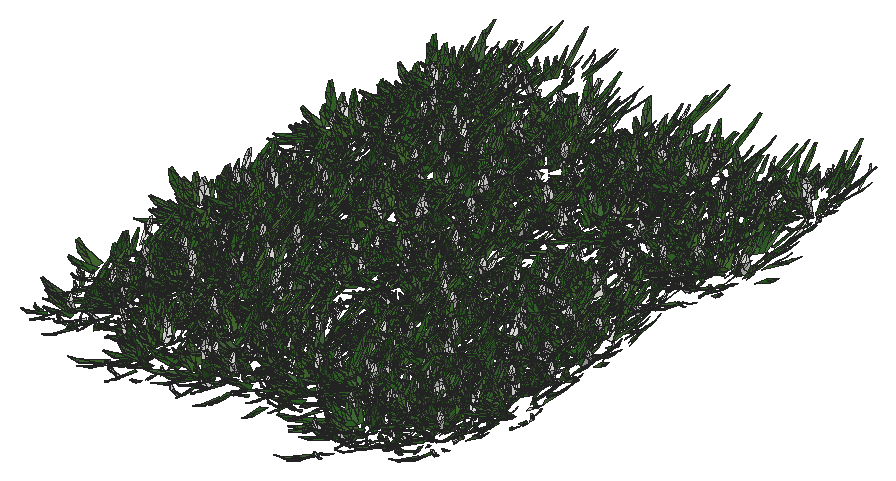
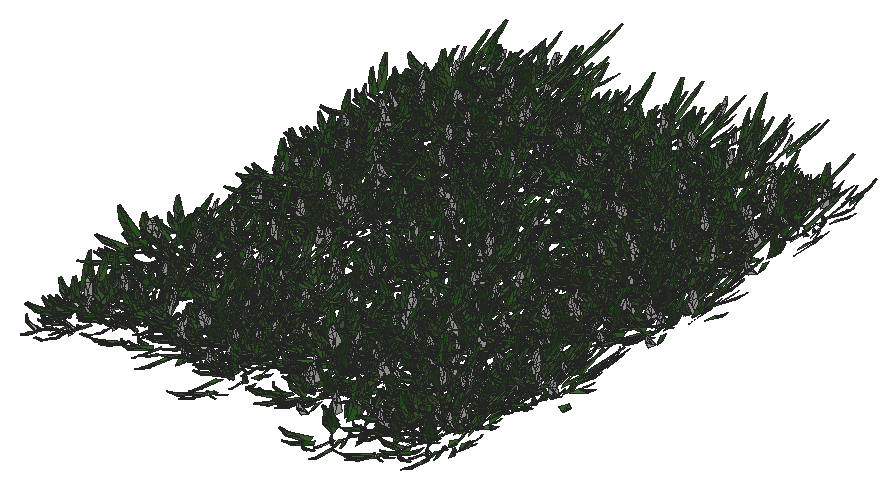
# SketchUp Ruby script. Lengths in inches.
U = 1.inch
M = Sketchup.active_model
def pt(a) = Geom::Point3d.new(a.map { |v| v * U })
def face(e, loops, mat)
  f = e.add_face(loops[0].map { |a| pt(a) })
  loops[1..].each { |l| e.add_face(l.map { |a| pt(a) }).erase! }
  f.material = f.back_material = mat if mat
  f
end
# faces: each face lists its corners as indices into pts; further lists are holes
def faces(e, pts, list, mat = nil) = list.each { |f| face(e, (f[0].is_a?(Array) ? f : [f]).map { |l| l.map { |i| pts[i] } }, mat) }
# xy, xz, yz: faces in a plane at the given z, y or x. An outline is a flat list of corners, or four numbers for a rectangle; further outlines are holes
def ring(l) = l.size == 4 ? [[l[0], l[1]], [l[2], l[1]], [l[2], l[3]], [l[0], l[3]]] : l.each_slice(2).to_a
def flat(e, list, mat, &to3) = list.each { |f| face(e, (f[0].is_a?(Array) ? f : [f]).map { |l| ring(l).map { |u, v| to3.(u, v) } }, mat) }
def xy(e, z, list, mat = nil) = flat(e, list, mat) { |x, y| [x, y, z] }
def xz(e, y, list, mat = nil) = flat(e, list, mat) { |x, z| [x, y, z] }
def yz(e, x, list, mat = nil) = flat(e, list, mat) { |y, z| [x, y, z] }
def lines(e, pts, list) = list.each { |a, b| e.add_line(pt(pts[a]), pt(pts[b])) }
# prism: a flat outline (further loops are holes) pulled along v
def prism(e, loops, v, mat = nil)
  f = face(e, loops, mat); d = Geom::Vector3d.new(v.map { |x| x * U })
  f.pushpull(f.normal.samedirection?(d) ? d.length : -d.length)
end
def box(e, o, s, mat = nil) = prism(e, [[o, [o[0] + s[0], o[1], o[2]], [o[0] + s[0], o[1] + s[1], o[2]], [o[0], o[1] + s[1], o[2]]]], [0, 0, s[2]], mat)
def at(x, y, z, deg = 0) = Geom::Transformation.translation(pt([x, y, z])) * Geom::Transformation.rotation(ORIGIN, Z_AXIS, deg.degrees)
def axes(o, x, y, z) = Geom::Transformation.new([*x, 0, *y, 0, *z, 0, *pt(o).to_a, 1])
def part(name) = M.definitions.add(name)
# library, detail: a bought-in or finely detailed component or shape, given as its bounding box
def library(name, o, s) = part(name).tap { |d| box(d.entities, o, s) }
def detail(e, o, s) = box(e.add_group.entities, o, s)
def put(e, d, t, mat = nil) = e.add_instance(d, t).tap { |i| i.material = mat if mat }
def group(e, t, mat = nil) = e.add_group.tap { |g| g.transformation = t; g.material = mat if mat }.entities
root = M.entities
M.materials.add("Material10").color = [48, 90, 38]
M.materials.add("Material11").color = [68, 110, 48]
M.materials.add("Material12").color = [48, 90, 48]
M.materials.add("Material13").color = [58, 110, 58]
M.materials.add("Material14").color = [58, 90, 38]
M.materials.add("Material15").color = [68, 100, 58]
M.materials.add("Material16").color = [48, 100, 38]
M.materials.add("Material9").color = [68, 110, 58]
c1 = part("grass00")
p = [[-0.6875,0.15,0],[-0.56,0.08,5.52],[-0.04,0.03,2.76],[0.48,-0.02,0],[0.35,-0.02,5.52],[-0.1,-0.14,5.52],
  [-0.12,0.65,8.37],[-0.42,0.65,8.37]]
faces(c1.entities,p,[[0,1,2,3],[3,2,4],[1,5,2],[5,4,2],[1,6,5],[4,5,6],[7,6,1]])
c2 = part("Group16\#1")
put(c2.entities,c1,axes([1.44,-0.61,-0.01],[0.05352,0.12609,0],[-0.10704,0.04543,0.07239],[0.06664,-0.02828,0.11628]),"Material12")
put(c2.entities,c1,axes([0.76,-0.15,-0.01],[0.04676,0.24062,0],[-0.23162,0.04501,0.06642],[0.0652,-0.01267,0.23595]),"Material9")
put(c2.entities,c1,axes([0.79,0.01,-0.01],[-0.00606,0.34651,0],[-0.34381,-0.00602,0.0432],[0.04319,0.00076,0.34386]))
put(c2.entities,c1,axes([1,0.23,-0.01],[-0.07192,0.31144,0],[-0.28722,-0.06632,0.1236],[0.12043,0.02781,0.29478]),"Material11")
put(c2.entities,c1,axes([1.66,0.77,-0.01],[-0.13828,0.29651,0],[-0.21551,-0.1005,0.22471],[0.20365,0.09498,0.23779]),"Material16")
put(c2.entities,c1,axes([0.6875,0.52,-0.01],[-0.18126,0.24051,0],[-0.22746,-0.17142,0.09788],[0.07817,0.05891,0.28481]),"Material11")
put(c2.entities,c1,axes([0.68,0.78,-0.01],[-0.215,0.18688,0],[-0.12385,-0.14248,0.21334],[0.13995,0.16101,0.18878]),"Material9")
put(c2.entities,c1,axes([0.56,1,-0.01],[-0.13756,0.07624,0],[-0.06159,-0.11112,0.0927],[0.04494,0.08108,0.12705]),"Material11")
put(c2.entities,c1,axes([0.2,0.64,-0.01],[-0.23729,0.07254,0],[-0.05711,-0.18681,0.153],[0.04473,0.14632,0.19535]),"Material16")
put(c2.entities,c1,axes([0.0625,0.72,-0.01],[-0.28874,0.02525,0],[-0.02179,-0.24916,0.14647],[0.01276,0.14591,0.25012]),"Material9")
put(c2.entities,c1,axes([-0.08,0.62,-0.01],[-0.34089,-0.04187,0],[0.03255,-0.26504,0.216],[-0.02633,0.21439,0.26703]),"Material16")
put(c2.entities,c1,axes([-0.34,0.98,-0.01],[-0.14314,-0.0493,0],[0.04397,-0.12769,0.06843],[-0.02228,0.0647,0.13505]),"Material16")
put(c2.entities,c1,axes([-0.87,1.45,-0.01],[-0.23488,-0.14114,0],[0.13761,-0.22901,0.06087],[-0.03135,0.05217,0.26717]))
put(c2.entities,c1,axes([-0.72,0.77,-0.01],[-0.14208,-0.13251,0],[0.07209,-0.0773,0.16301],[-0.11118,0.11922,0.1057]),"Material16")
put(c2.entities,c1,axes([-0.62,0.43,-0.01],[-0.14845,-0.21203,0],[0.18654,-0.13061,0.12304],[-0.10079,0.07057,0.22772]),"Material9")
put(c2.entities,c1,axes([-0.68,0.29,-0.01],[-0.13639,-0.32136,0],[0.31723,-0.13464,0.05579],[-0.05136,0.0218,0.34462]),"Material10")
put(c2.entities,c1,axes([-0.64,0.125,-0.01],[-0.0458,-0.23569,0],[0.22124,-0.043,0.08276],[-0.08124,0.01579,0.22538]),"Material13")
put(c2.entities,c1,axes([-1.6,-0.03,-0.01],[0.00576,-0.32897,0],[0.27526,0.00482,0.18018],[-0.18015,-0.00315,0.2753]),"Material11")
put(c2.entities,c1,axes([-1.36,-0.31,-0.01],[0.05718,-0.24765,0],[0.18172,0.04196,0.17267],[-0.16825,-0.03885,0.1865]),"Material16")
put(c2.entities,c1,axes([-1.54,-0.72,-0.01],[0.06537,-0.14017,0],[0.13555,0.06321,0.03939],[-0.0357,-0.01665,0.14956]))
put(c2.entities,c1,axes([-1.19,-0.9,-0.01],[0.09597,-0.12735,0],[0.11214,0.08451,0.07557],[-0.06035,-0.04548,0.14042]),"Material15")
put(c2.entities,c1,axes([-0.47,-0.54,-0.01],[0.11588,-0.10072,0],[0.0618,0.0711,0.12124],[-0.07953,-0.0915,0.0942]))
put(c2.entities,c1,axes([-0.47,-0.84,-0.01],[0.11927,-0.0661,0],[0.06603,0.11913,0.00646],[-0.00313,-0.00565,0.13621]),"Material11")
put(c2.entities,c1,axes([-0.38,-1.24,-0.01],[0.28037,-0.08571,0],[0.0618,0.20215,0.20315],[-0.05939,-0.19428,0.21139]),"Material15")
put(c2.entities,c1,axes([-0.06,-0.66,-0.01],[0.22719,-0.01987,0],[0.01247,0.14255,0.17758],[-0.01547,-0.17691,0.1431]),"Material14")
put(c2.entities,c1,axes([0.11,-0.89,-0.01],[0.14882,0.01828,0],[-0.01058,0.08611,0.12229],[0.01491,-0.12138,0.08676]),"Material12")
put(c2.entities,c1,axes([0.25,-0.72,-0.01],[0.20481,0.07053,0],[-0.06206,0.18022,0.10291],[0.03351,-0.0973,0.1906]),"Material12")
put(c2.entities,c1,axes([0.85,-1.42,-0.01],[0.16481,0.09904,0],[-0.09472,0.15762,0.05616],[0.02893,-0.04814,0.18389]),"Material11")
put(c2.entities,c1,axes([1.01,-1.09,-0.01],[0.21858,0.20385,0],[-0.17495,0.1876,0.15339],[0.10462,-0.11218,0.25652]),"Material16")
put(c2.entities,c1,axes([1.01,-0.71,-0.01],[0.08733,0.12473,0],[-0.06445,0.04512,0.13037],[0.1068,-0.07477,0.07867]),"Material12")
c3 = part("Group15\#1")
put(c3.entities,c2,at(0,0,0))
c4 = part("3darcstudiotree_grass00\#1")
put(c4.entities,c3,at(0,0,0))
put(root,c4,axes([827.38,626.97,12.99],[-2.37423,5.49168,0],[-1.9202,-4.33781,-0.03007],[-0.11385,-0.2572,1.97134]))
put(root,c4,axes([873.03,627.38,12.99],[0.43076,7.5469,0],[-2.49885,0.74527,-0.03746],[-0.18093,0.05396,1.68385]))
put(root,c4,axes([877.48,630.32,12.99],[2.41678,2.99983,0],[-1.2331,5.19091,-0.03457],[-0.08948,0.37667,1.92264]))
put(root,c4,axes([838.15,629.06,12.99],[-2.83663,1.42991,0],[-0.68383,-7.08843,-0.02531],[-0.02216,-0.2297,1.77094]))
put(root,c4,axes([824.06,630.47,12.99],[1.45141,7.05761,0],[-2.63622,2.83281,-0.03464],[-0.13976,0.15018,1.78143]))
put(root,c4,axes([851.625,633.5,12.99],[-0.02714,-5.82312,0],[3.4571,-0.0842,-0.05216],[0.14988,-0.00365,1.36288]))
put(root,c4,axes([803.71,634.1,12.99],[0.90647,-5.26217,0],[2.79568,2.51641,-0.0431],[0.13449,0.12105,1.38217]))
put(root,c4,axes([808.97,633.48,12.99],[2.65153,2.38197,0],[-1.03238,6.00489,-0.02634],[-0.03943,0.22937,1.58474]))
put(root,c4,axes([842.07,635.41,12.99],[0.95151,-7.55802,0],[3.30412,2.17354,-0.04991],[0.1976,0.12999,1.94306]))
put(root,c4,axes([870.84,632.96,12.99],[-3.13855,-0.88162,0],[0.39114,-7.27583,-0.04768],[0.0198,-0.36827,1.49744]))
put(root,c4,axes([843.74,633.08,12.99],[-1.41677,7.11189,0],[-2.22403,-2.31505,-0.04508],[-0.16224,-0.16888,1.32557]))
put(root,c4,axes([824.7,635.18,12.99],[-0.89079,-5.45923,0],[2.93999,-2.50666,-0.0406],[0.16325,-0.13919,1.84742]))
put(root,c4,axes([882.71,635.9,12.99],[2.96033,-0.5202,0],[0.24057,7.15334,-0.03486],[0.01046,0.311,1.68524]))
put(root,c4,axes([836.04,637.33,12.99],[0.52554,-6.14252,0],[3.42043,1.52912,-0.06032],[0.17465,0.07808,1.41053]))
put(root,c4,axes([820.39,637.29,12.99],[0.17649,-6.6496,0],[3.22338,0.44704,-0.04584],[0.13578,0.01883,1.3146]))
put(root,c4,axes([861.75,637.18,12.99],[2.53106,4.3429,0],[-1.85243,5.64117,-0.02233],[-0.06236,0.18989,1.9689]))
put(root,c4,axes([856.68,636.47,12.99],[-2.58773,4.03605,0],[-1.59912,-5.35732,-0.04776],[-0.11569,-0.38757,1.6727]))
put(root,c4,axes([874.8125,638.46,12.99],[1.38554,6.71769,0],[-2.60751,2.81016,-0.03917],[-0.16088,0.17338,1.79585]))
put(root,c4,axes([866.72,638.83,12.99],[0.12549,7.79346,0],[-3.40251,0.28627,-0.03073],[-0.09784,0.00823,1.48809]))
put(root,c4,axes([886.75,638.65,12.99],[-0.79908,7.12585,0],[-3.17807,-1.86218,-0.05431],[-0.19695,-0.1154,1.6847]))
put(root,c4,axes([836.7,642.28,12.99],[2.73963,-0.34023,0],[0.14501,6.10118,-0.02262],[0.0054,0.22718,1.6131]))
put(root,c4,axes([811.9,639.8,12.99],[-1.74597,5.76407,0],[-2.15705,-3.41407,-0.03104],[-0.12661,-0.20039,1.78553]))
put(root,c4,axes([851.64,642.82,12.99],[-0.39937,-7.02713,0],[2.45826,-0.73001,-0.04034],[0.17351,-0.05153,1.47504]))
put(root,c4,axes([832.96,643.67,12.99],[-1.43376,-4.96537,0],[2.07832,-3.13575,-0.03406],[0.14408,-0.21739,1.73123]))
put(root,c4,axes([862.18,644.98,12.99],[2.57457,-3.51757,0],[1.66433,6.36512,-0.05659],[0.10752,0.4112,1.64805]))
put(root,c4,axes([810.82,642.92,12.99],[-2.82662,-1.37215,0],[0.64948,-6.99095,-0.02543],[0.0198,-0.2131,1.60712]))
put(root,c4,axes([847.42,645.02,12.99],[-0.04441,-5.91504,0],[3.02597,-0.11872,-0.0405],[0.18434,-0.00723,1.89003]))
put(root,c4,axes([881.23,642.45,12.99],[-3.19545,2.75579,0],[-1.21799,-7.37964,-0.03096],[-0.04152,-0.25159,1.79846]))
put(root,c4,axes([846.15,643.85,12.99],[-0.34531,6.17385,0],[-3.32473,-0.97165,-0.0277],[-0.11233,-0.03283,1.87956]))
put(root,c4,axes([878.14,645.06,12.99],[1.84367,4.1672,0],[-1.70839,3.94941,-0.02576],[-0.1024,0.23673,1.88472]))
put(root,c4,axes([825.89,648.15,12.99],[1.25304,-5.40337,0],[2.85201,3.45587,-0.01977],[0.07044,0.08535,1.78562]))
put(root,c4,axes([886.66,647,12.99],[1.945,3.95778,0],[-2.10927,5.41631,-0.03405],[-0.08629,0.22159,1.65877]))
put(root,c4,axes([802.61,648.01,12.99],[3.06395,1.36265,0],[-0.61914,7.27433,-0.03864],[-0.03074,0.36119,1.85268]))
put(root,c4,axes([809.37,648.66,12.99],[2.23298,-4.95504,0],[1.79016,4.21537,-0.02978],[0.08432,0.19856,1.43312]))
put(root,c4,axes([857.9375,647.72,12.99],[-1.4711,-5.8297,0],[2.67186,-3.52304,-0.05686],[0.15267,-0.2013,1.31145]))
put(root,c4,axes([815.91,646.11,12.99],[-0.90996,6.13703,0],[-2.95759,-2.29145,-0.05878],[-0.18054,-0.13988,1.38915]))
put(root,c4,axes([868.14,647.99,12.99],[-2.61801,-2.5298,0],[1.19759,-6.4759,-0.0473],[0.06262,-0.3386,1.43445]))
put(root,c4,axes([865.81,649.17,12.99],[2.88934,4.27674,0],[-1.72566,6.09181,-0.02279],[-0.05355,0.18905,1.88252]))
put(root,c4,axes([845.39,653.56,12.99],[-0.34485,-6.99494,0],[2.81083,-0.72408,-0.02839],[0.09584,-0.02469,1.31807]))
put(root,c4,axes([876.6,652.99,12.99],[-1.44959,-4.55091,0],[2.53951,-4.22671,-0.06067],[0.206,-0.34286,1.80988]))
put(root,c4,axes([890.19,652.17,12.99],[-2.81566,3.68421,0],[-1.29367,-5.16611,-0.03218],[-0.07418,-0.29624,1.65786]))
put(root,c4,axes([856.61,653.59,12.99],[1.64625,5.68783,0],[-2.83649,4.28977,-0.02773],[-0.07489,0.11325,1.51065]))
put(root,c4,axes([864.83,652.91,12.99],[1.37491,7.18474,0],[-2.38597,2.3858,-0.02724],[-0.10498,0.10497,1.50258]))
put(root,c4,axes([884.38,655.29,12.99],[0.34051,-7.93068,0],[3.2082,0.71976,-0.05803],[0.17098,0.03836,1.30918]))
put(root,c4,axes([837.18,654.88,12.99],[-0.60636,-6.78227,0],[3.22523,-1.50669,-0.03636],[0.12915,-0.06034,1.63697]))
put(root,c4,axes([816.36,656.6,12.99],[0.27663,-7.59076,0],[2.72705,0.5193,-0.04948],[0.23162,0.04411,1.76318]))
put(root,c4,axes([811.54,657.04,12.99],[2.21176,-3.78503,0],[1.87777,5.73344,-0.01707],[0.04665,0.14244,1.96039]))
put(root,c4,axes([833.02,655.55,12.99],[2.89688,4.51213,0],[-1.74859,5.86599,-0.06012],[-0.10731,0.36,1.3502]))
put(root,c4,axes([827.35,657.01,12.99],[2.46753,-0.03989,0],[0.02228,7.20222,-0.0442],[0.00097,0.31246,1.33678]))
put(root,c4,axes([807.8,656.56,12.99],[1.88814,4.33242,0],[-2.29446,5.22502,-0.03194],[-0.06946,0.15819,1.36388]))
put(root,c4,axes([873.38,655.6875,12.99],[-2.65419,1.56606,0],[-0.68524,-6.06832,-0.03018],[-0.03978,-0.35226,1.98332]))
put(root,c4,axes([825.84,657.81,12.99],[-1.80112,-5.98247,0],[2.61779,-4.11815,-0.05298],[0.14778,-0.23247,1.4759]))
put(root,c4,axes([819.19,658.38,12.99],[1.66345,4.98196,0],[-1.98596,3.46486,-0.04536],[-0.20249,0.35328,1.92466]))
put(root,c4,axes([882.75,661.34,12.99],[2.26154,-4.66794,0],[1.96985,4.98675,-0.04418],[0.12328,0.3121,1.67893]))
put(root,c4,axes([855.9375,661.76,12.99],[0.70019,-6.81469,0],[3.11491,1.67232,-0.04288],[0.16211,0.08703,1.70449]))
put(root,c4,axes([878.21,661.8125,12.99],[3.25532,2.0612,0],[-0.92871,7.66407,-0.02222],[-0.02404,0.19841,1.93436]))
put(root,c4,axes([807.79,663.53,12.99],[0.74589,-6.35213,0],[3.04859,1.87051,-0.05256],[0.1865,0.11443,1.59089]))
put(root,c4,axes([853.92,662.66,12.99],[-1.88477,-4.86997,0],[2.03275,-4.11074,-0.02762],[0.09343,-0.18895,1.68176]))
put(root,c4,axes([823.78,661.02,12.99],[-2.26827,5.60399,0],[-2.14024,-4.52652,-0.0352],[-0.10497,-0.222,1.62511]))
put(root,c4,axes([832.97,664.07,12.99],[0.44453,-7.27791,0],[2.48239,0.79227,-0.0384],[0.16951,0.0541,1.53253]))
put(root,c4,axes([864.75,665.3,12.99],[2.26347,-2.39045,0],[1.05596,5.22453,-0.0238],[0.05531,0.27364,1.9133]))
put(root,c4,axes([820.26,666.875,12.99],[-0.09218,-7.71818,0],[3.4905,-0.21784,-0.06757],[0.24622,-0.01537,1.74608]))
put(root,c4,axes([888.66,667.875,12.99],[0.94107,-5.1818,0],[2.54729,2.41728,-0.03248],[0.12784,0.12131,1.61223]))
put(root,c4,axes([884.36,666.12,12.99],[0.83936,5.86752,0],[-2.87512,2.14908,-0.05705],[-0.19968,0.14925,1.52794]))
put(root,c4,axes([868.13,666.78,12.99],[0.90786,5.26282,0],[-2.43808,2.19763,-0.04901],[-0.20896,0.18835,1.64754]))
put(root,c4,axes([839.23,666.4,12.99],[-0.71302,5.98674,0],[-3.33162,-2.07336,-0.06593],[-0.21513,-0.13388,1.60187]))
put(root,c4,axes([815.01,667.57,12.99],[-2.94486,-2.55627,0],[1.09203,-6.57349,-0.04397],[0.07134,-0.42941,1.92843]))
put(root,c4,axes([814.85,671.08,12.99],[2.86272,-3.15992,0],[1.14707,5.43,-0.04306],[0.10093,0.47778,1.95064]))
put(root,c4,axes([803.48,673.38,12.99],[-1.55839,-6.34101,0],[2.59431,-3.33153,-0.0488],[0.13834,-0.17766,1.32723]))
put(root,c4,axes([869.1,673.41,12.99],[3.15436,2.86223,0],[-1.04743,6.03166,-0.04113],[-0.05358,0.30857,1.37498]))
put(root,c4,axes([856.06,674.46,12.99],[3.0711,-2.53194,0],[1.13742,7.20885,-0.06016],[0.06772,0.42923,1.52593]))
put(root,c4,axes([853.08,671.91,12.99],[0.4786,7.36211,0],[-2.65372,0.90143,-0.03328],[-0.1372,0.0466,1.53387]))
put(root,c4,axes([833.09,672.64,12.99],[-1.1272,5.38552,0],[-2.68054,-2.93158,-0.02774],[-0.08686,-0.09499,1.41462]))
put(root,c4,axes([820.11,675.625,12.99],[2.45785,-3.50695,0],[1.56675,5.73761,-0.03499],[0.08624,0.31583,1.88939]))
put(root,c4,axes([800.61,672.56,12.99],[-2.4779,4.13156,0],[-1.88431,-5.90511,-0.03459],[-0.08564,-0.26838,1.84283]))
put(root,c4,axes([884.97,674.7,12.99],[-2.03841,-5.5397,0],[2.33633,-4.49203,-0.04595],[0.14709,-0.2828,1.75181]))
put(root,c4,axes([847.71,675.4,12.99],[-1.02657,-6.63243,0],[2.63813,-2.13361,-0.03351],[0.13906,-0.11247,1.68972]))
put(root,c4,axes([880.73,675.4375,12.99],[2.85064,3.12184,0],[-1.37003,6.53683,-0.04599],[-0.06237,0.29759,1.36526]))
put(root,c4,axes([813.26,674.75,12.99],[-1.7901,4.03362,0],[-2.31104,-5.35914,-0.05994],[-0.14127,-0.32759,1.51606]))
put(root,c4,axes([877.75,677.02,12.99],[-2.78696,-4.07137,0],[1.74298,-6.23428,-0.05584],[0.1313,-0.46963,1.93872]))
put(root,c4,axes([841.09,675.77,12.99],[-0.44832,7.66632,0],[-2.66418,-0.81408,-0.04319],[-0.21735,-0.06641,1.87209]))
put(root,c4,axes([888.33,676.14,12.99],[-0.50033,7.82831,0],[-2.68587,-0.89697,-0.03578],[-0.12749,-0.04258,1.34076]))
put(root,c4,axes([853.51,681.18,12.99],[1.57074,-6.53994,0],[2.45907,3.08606,-0.02765],[0.09685,0.12154,1.53783]))
put(root,c4,axes([800.5,680.89,12.99],[2.292,2.04989,0],[-1.23841,7.23528,-0.03882],[-0.04731,0.27643,1.55956]))
put(root,c4,axes([804.64,679.9,12.99],[2.06212,4.33403,0],[-1.95148,4.85168,-0.04265],[-0.13868,0.34479,1.90027]))
put(root,c4,axes([811.71,681.33,12.99],[3.03896,2.02803,0],[-0.78091,6.11445,-0.03197],[-0.03224,0.25246,1.37583]))
put(root,c4,axes([845.47,682.15,12.99],[-1.66013,-5.04205,0],[2.03322,-3.49804,-0.02546],[0.11325,-0.19484,1.94365]))
put(root,c4,axes([861.51,683.45,12.99],[-1.40686,-5.29098,0],[2.17321,-3.0194,-0.04312],[0.20287,-0.28186,1.92045]))
put(root,c4,axes([807.55,681.75,12.99],[-1.86769,6.5308,0],[-2.31191,-3.45474,-0.05029],[-0.22101,-0.33026,1.98932]))
put(root,c4,axes([840.6875,681.93,12.99],[-1.11152,5.01709,0],[-2.60811,-3.01922,-0.03106],[-0.09152,-0.10595,1.32443]))
put(root,c4,axes([876.5,685.39,12.99],[2.50536,-3.77628,0],[1.7468,6.05555,-0.02666],[0.05017,0.17392,1.48784]))
put(root,c4,axes([835.81,684.9,12.99],[0.10771,-5.80364,0],[3.36464,0.32628,-0.04061],[0.15016,0.01456,1.70991]))
put(root,c4,axes([869.12,684.42,12.99],[2.76122,2.41363,0],[-1.00808,6.02601,-0.02441],[-0.04439,0.26536,1.97124]))
put(root,c4,axes([815.61,682.9,12.99],[0.08869,5.99183,0],[-3.3201,0.25679,-0.06181],[-0.23999,0.01856,1.77032]))
put(root,c4,axes([865.64,684.18,12.99],[2.0459,3.39209,0],[-1.4292,4.50419,-0.02439],[-0.06896,0.21732,1.60766]))
put(root,c4,axes([884.62,685.98,12.99],[1.61595,-5.02508,0],[2.65261,4.45721,-0.0227],[0.06517,0.10951,1.60931]))
put(root,c4,axes([820.16,685.43,12.99],[2.14992,4.87555,0],[-1.93384,4.45578,-0.02475],[-0.07543,0.17381,1.62992]))
put(root,c4,axes([829.37,686.05,12.99],[-1.84879,4.09416,0],[-2.20659,-5.20654,-0.02879],[-0.08101,-0.19114,1.7592]))
put(root,c4,axes([868.19,689.42,12.99],[1.50147,-4.51305,0],[2.75817,4.79483,-0.04371],[0.103,0.17905,1.40723]))
put(root,c4,axes([808.43,689.34,12.99],[2.99349,3.64239,0],[-1.51439,6.5033,-0.02998],[-0.06312,0.27104,1.98098]))
put(root,c4,axes([853.7,690.78,12.99],[1.67224,-5.15475,0],[2.54088,4.30706,-0.03781],[0.10077,0.17081,1.4396]))
put(root,c4,axes([878,689.6875,12.99],[-2.61547,4.64016,0],[-1.917,-5.64604,-0.03049],[-0.0757,-0.22297,1.73706]))
put(root,c4,axes([811.19,692.49,12.99],[2.86639,-1.64322,0],[0.59398,5.414,-0.03452],[0.04673,0.4259,1.86367]))
put(root,c4,axes([845.42,693.34,12.99],[1.0963,-5.09622,0],[2.34462,2.63547,-0.04022],[0.20118,0.22614,1.99791]))
put(root,c4,axes([815.07,693.4,12.99],[2.36507,1.59346,0],[-0.92066,7.14012,-0.04213],[-0.03804,0.29502,1.42653]))
put(root,c4,axes([825.87,691.88,12.99],[0.87745,5.33249,0],[-2.63208,2.26306,-0.04913],[-0.21681,0.18641,1.81865]))
put(root,c4,axes([831.61,694.24,12.99],[3.12392,-1.43629,0],[0.60263,6.84877,-0.02659],[0.019,0.21589,1.51897]))
put(root,c4,axes([836.59,695.98,12.99],[-3.43263,0.08415,0],[-0.03476,-7.40959,-0.01941],[-0.0009,-0.19244,1.92834]))
put(root,c4,axes([823.75,698.99,12.99],[-2.64349,-4.9904,0],[2.06968,-5.72864,-0.02974],[0.05736,-0.15877,1.35064]))
put(root,c4,axes([846.1,700.71,12.99],[-1.29606,-6.58218,0],[2.79639,-2.87713,-0.04331],[0.17728,-0.1824,1.88835]))
put(root,c4,axes([882.25,699.85,12.99],[-2.35958,-2.55628,0],[1.2462,-6.01059,-0.03887],[0.06114,-0.29487,1.46596]))
put(root,c4,axes([867.92,699.35,12.99],[-2.90669,-0.11289,0],[0.05546,-7.46174,-0.03595],[0.00227,-0.30532,1.66434]))
put(root,c4,axes([808.12,701.78,12.99],[-0.60445,-5.98981,0],[2.85983,-1.50796,-0.03351],[0.12965,-0.06837,1.59864]))
put(root,c4,axes([866.57,702.47,12.99],[1.32603,-5.43218,0],[2.35375,3.00222,-0.05199],[0.17435,0.22238,1.41973]))
put(root,c4,axes([849.65,702.31,12.99],[-0.34945,-6.41359,0],[3.29737,-0.93878,-0.06365],[0.26262,-0.07477,1.89522]))
put(root,c4,axes([836.58,702.92,12.99],[3.24619,-1.29562,0],[0.60028,7.85878,-0.04063],[0.02133,0.2792,1.46079]))
put(root,c4,axes([817.3125,702.21,12.99],[2.9897,1.23836,0],[-0.53674,6.77093,-0.0513],[-0.03431,0.4328,1.54883]))
put(root,c4,axes([873.37,708.86,12.99],[0.78909,-6.29385,0],[2.78303,1.82319,-0.03571],[0.16951,0.11105,1.9611]))
put(root,c4,axes([824.11,709.98,12.99],[2.9346,0.12145,0],[-0.0596,7.52541,-0.04973],[-0.00379,0.47813,1.89995]))
put(root,c4,axes([828.06,709.92,12.99],[-2.35089,-5.37346,0],[2.18019,-4.98399,-0.05204],[0.15418,-0.35246,1.77215]))
put(root,c4,axes([832.2,710.4,12.99],[2.7136,4.20157,0],[-1.93348,6.52498,-0.02464],[-0.05793,0.19551,1.98292]))
put(root,c4,axes([856.31,711.43,12.99],[1.2386,-5.85682,0],[2.60656,2.88033,-0.03335],[0.12099,0.1337,1.60043]))
put(root,c4,axes([835.53,712.3,12.99],[2.38444,-4.3099,0],[1.98898,5.74982,-0.01988],[0.05504,0.15911,1.96304]))
put(root,c4,axes([878.2,712.34,12.99],[1.48211,-4.9105,0],[2.2179,3.49787,-0.0362],[0.15554,0.24531,1.92943]))
put(root,c4,axes([807.51,710.03,12.99],[-2.03485,3.55217,0],[-1.9623,-5.87366,-0.0597],[-0.15796,-0.47281,1.93343]))
put(root,c4,axes([815.57,711.1875,12.99],[2.24922,5.09487,0],[-2.43674,5.62099,-0.05903],[-0.16095,0.37127,1.83956]))
put(root,c4,axes([889.07,711.19,12.99],[0.22264,6.72647,0],[-2.77145,0.47932,-0.04286],[-0.15966,0.02761,1.42447]))
put(root,c4,axes([800.58,711.16,12.99],[-1.85033,5.34695,0],[-2.41629,-4.36916,-0.0328],[-0.0807,-0.14591,1.32564]))
put(root,c4,axes([819.34,714.47,12.99],[1.61599,-5.9307,0],[2.54954,3.62995,-0.04551],[0.1569,0.22339,1.67334]))
put(root,c4,axes([803.17,713.11,12.99],[-2.64737,-1.79319,0],[0.79517,-6.13413,-0.05017],[0.05725,-0.44168,1.54202]))
put(root,c4,axes([850.24,712.67,12.99],[-2.58987,2.35124,0],[-1.01273,-5.82881,-0.04199],[-0.06939,-0.39938,1.68502]))
put(root,c4,axes([861.01,712.94,12.99],[1.07852,7.26808,0],[-3.04885,2.36401,-0.04327],[-0.16331,0.12663,1.7601]))
put(root,c4,axes([880.46,713.43,12.99],[-0.17715,6.01345,0],[-2.92707,-0.45055,-0.04305],[-0.19081,-0.02937,1.78778]))
put(root,c4,axes([885.61,714.66,12.99],[-2.60665,-0.08038,0],[0.03801,-6.44071,-0.03579],[0.00201,-0.34028,1.60809]))
put(root,c4,axes([852.31,718.89,12.99],[2.8606,-1.47641,0],[0.58856,5.95866,-0.03599],[0.02858,0.28937,1.32194]))
put(root,c4,axes([889.68,719.99,12.99],[2.59192,-4.60907,0],[2.08003,6.11197,-0.05588],[0.12334,0.36243,1.67045]))
put(root,c4,axes([804.875,718.25,12.99],[-3.0163,-1.47855,0],[0.59519,-6.34453,-0.03168],[0.02497,-0.26619,1.46389]))
put(root,c4,axes([868.94,719.5625,12.99],[-2.20882,-2.34735,0],[1.08701,-5.34464,-0.04575],[0.08742,-0.42982,1.60296]))
put(root,c4,axes([820.52,722.05,12.99],[0.19957,-5.95289,0],[3.02318,0.52959,-0.05496],[0.25303,0.04433,1.9204]))
put(root,c4,axes([863.88,720.6,12.99],[-2.45449,-3.83246,0],[1.97739,-6.6173,-0.03279],[0.06523,-0.21828,1.69581]))
put(root,c4,axes([809.53,722.06,12.99],[2.53927,0.89631,0],[-0.42559,6.30014,-0.03647],[-0.02284,0.33806,1.56991]))
put(root,c4,axes([861.64,722.86,12.99],[-1.57231,-4.70852,0],[2.08644,-3.64053,-0.04177],[0.12625,-0.22029,1.36919]))
put(root,c4,axes([831.11,722.66,12.99],[-2.40394,-3.68349,0],[1.73965,-5.93243,-0.05337],[0.10993,-0.37486,1.58535]))
put(root,c4,axes([880.18,721.43,12.99],[-0.64404,7.10182,0],[-2.73222,-1.29469,-0.02464],[-0.11324,-0.05366,1.79662]))
put(root,c4,axes([841.97,723.5625,12.99],[-1.6465,-4.6626,0],[2.03066,-3.74694,-0.02577],[0.08771,-0.16183,1.56591]))
put(root,c4,axes([841.88,726.62,12.99],[-1.94693,-6.6689,0],[2.23331,-3.40683,-0.04802],[0.18422,-0.28101,1.69851]))
put(root,c4,axes([828.24,726.98,12.99],[-0.51441,-5.52691,0],[2.84235,-1.38233,-0.04713],[0.18311,-0.08905,1.58351]))
put(root,c4,axes([838.09,727.42,12.99],[3.18471,-1.03299,0],[0.45579,7.3425,-0.05794],[0.03338,0.53766,1.82474]))
put(root,c4,axes([825.39,729.35,12.99],[2.49651,-0.13706,0],[0.07551,7.1869,-0.04057],[0.00302,0.28761,1.33829]))
put(root,c4,axes([815.02,731.07,12.99],[1.72838,-6.07507,0],[2.10062,3.12278,-0.04791],[0.20615,0.30647,1.76421]))
put(root,c4,axes([878.45,730.08,12.99],[1.80024,4.554,0],[-2.1186,4.37614,-0.0306],[-0.10808,0.22326,1.86488]))
put(root,c4,axes([851.86,729.54,12.99],[0.29428,6.45652,0],[-2.91969,0.69536,-0.02993],[-0.11943,0.02844,1.61572]))
put(root,c4,axes([813.1,730.4375,12.99],[-2.40459,-2.61484,0],[1.4124,-6.78672,-0.03826],[0.06667,-0.32036,1.82966]))
put(root,c4,axes([849.08,732.72,12.99],[2.66802,-2.4343,0],[1.01732,5.82611,-0.02611],[0.03697,0.21172,1.43783]))
put(root,c4,axes([805.42,730.25,12.99],[-1.55697,6.57624,0],[-2.85897,-3.53686,-0.04902],[-0.1708,-0.21129,1.76654]))
put(root,c4,axes([872.54,732.05,12.99],[-2.18505,-3.91292,0],[1.80202,-5.25808,-0.04081],[0.09193,-0.26823,1.46417]))
put(root,c4,axes([831.9,732.84,12.99],[-2.58866,-3.06213,0],[1.37567,-6.07673,-0.02021],[0.04336,-0.19154,1.91641]))
put(root,c4,axes([861.63,732.49,12.99],[-0.48235,6.2889,0],[-2.83089,-1.13452,-0.02601],[-0.10795,-0.04326,1.66111]))
put(root,c4,axes([807.18,732.41,12.99],[-1.26714,5.58392,0],[-2.7275,-3.23411,-0.04385],[-0.13065,-0.15492,1.41492]))
put(root,c4,axes([855.74,732.84,12.99],[-3.02063,2.52489,0],[-0.85096,-5.3195,-0.04181],[-0.05803,-0.36274,1.37365]))
put(root,c4,axes([864.23,733.26,12.99],[0.46247,7.80605,0],[-3.30246,1.02234,-0.03426],[-0.13155,0.04072,1.77113]))
put(root,c4,axes([812.98,736.46,12.99],[1.76669,-5.36868,0],[2.62675,4.51664,-0.05537],[0.14811,0.25467,1.50911]))
put(root,c4,axes([861.52,736.02,12.99],[2.92544,-0.50627,0],[0.21311,6.43449,-0.04662],[0.01528,0.46123,1.68074]))
put(root,c4,axes([836.55,735.99,12.99],[-1.47421,6.19673,0],[-2.44502,-3.03937,-0.03157],[-0.13088,-0.1627,1.80167]))
put(root,c4,axes([852.52,736.68,12.99],[0.13407,6.92871,0],[-2.85667,0.28883,-0.03464],[-0.13811,0.01396,1.56527]))
put(root,c4,axes([833.2,738.96,12.99],[2.56819,0.83776,0],[-0.45356,7.26526,-0.03434],[-0.01881,0.30137,1.70799]))
put(root,c4,axes([865.71,736.32,12.99],[-1.60829,7.10744,0],[-2.93798,-3.47381,-0.04288],[-0.1417,-0.16754,1.68813]))
put(root,c4,axes([816.25,737.42,12.99],[-1.2812,5.51986,0],[-2.73632,-3.31865,-0.05129],[-0.14301,-0.17344,1.34106]))
put(root,c4,axes([881.39,740.44,12.99],[1.91363,-5.42934,0],[2.07396,3.81959,-0.02709],[0.10464,0.19272,1.8123]))
put(root,c4,axes([872.95,740.3,12.99],[-0.3163,-5.80826,0],[3.29062,-0.93636,-0.05859],[0.23467,-0.06678,1.83593]))
put(root,c4,axes([857.93,738.54,12.99],[-3.42714,0.73903,0],[-0.23141,-5.60722,-0.02738],[-0.01245,-0.30164,1.63584]))
put(root,c4,axes([809.49,740.74,12.99],[-0.91585,-7.6115,0],[3.09106,-1.94343,-0.02011],[0.0867,-0.05451,1.9663]))
put(root,c4,axes([804.0625,740.97,12.99],[-1.97775,-4.21493,0],[2.06336,-5.05896,-0.04642],[0.11521,-0.28246,1.51042]))
put(root,c4,axes([848.04,742.1,12.99],[-0.66563,-7.53304,0],[3.00071,-1.38545,-0.03802],[0.15864,-0.07325,1.78771]))
put(root,c4,axes([885.36,742.46,12.99],[-2.24553,3.94119,0],[-1.85205,-5.51378,-0.05552],[-0.1324,-0.39417,1.63365]))
put(root,c4,axes([886.04,745.6875,12.99],[1.60808,-5.87724,0],[2.16221,3.09127,-0.0272],[0.11994,0.17148,1.81972]))
put(root,c4,axes([820.74,748.37,12.99],[-1.78661,-4.66535,0],[2.50848,-5.01953,-0.03006],[0.0857,-0.17149,1.73276]))
